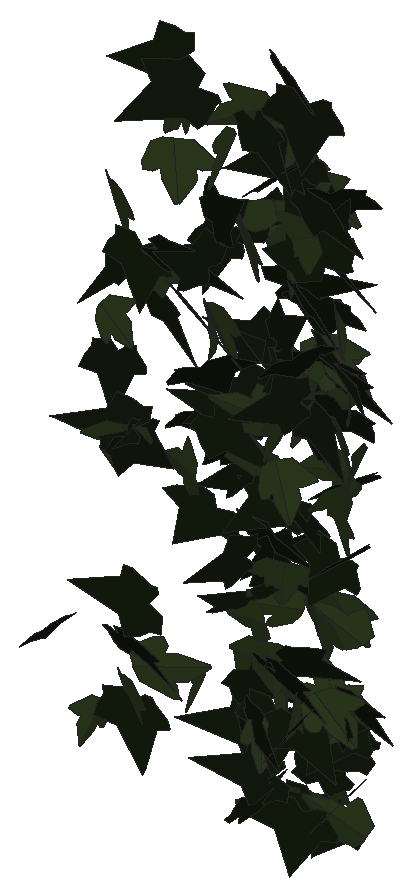
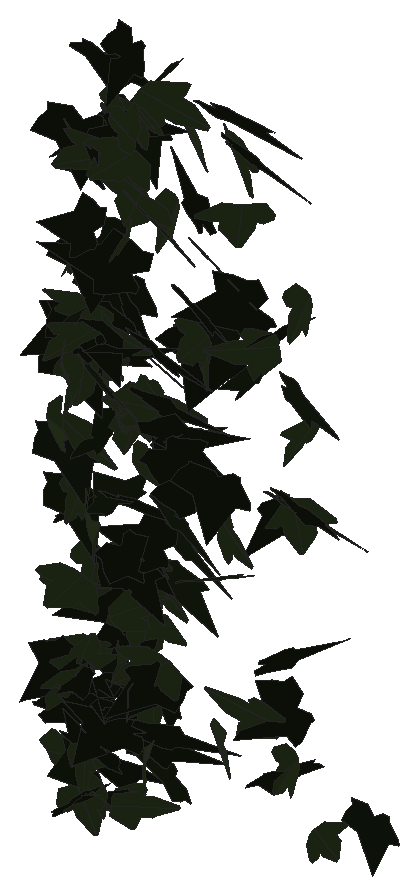
# SketchUp Ruby script. Lengths in inches.
U = 1.inch
M = Sketchup.active_model
def pt(a) = Geom::Point3d.new(a.map { |v| v * U })
def face(e, loops, mat)
  f = e.add_face(loops[0].map { |a| pt(a) })
  loops[1..].each { |l| e.add_face(l.map { |a| pt(a) }).erase! }
  f.material = f.back_material = mat if mat
  f
end
# faces: each face lists its corners as indices into pts; further lists are holes
def faces(e, pts, list, mat = nil) = list.each { |f| face(e, (f[0].is_a?(Array) ? f : [f]).map { |l| l.map { |i| pts[i] } }, mat) }
# xy, xz, yz: faces in a plane at the given z, y or x. An outline is a flat list of corners, or four numbers for a rectangle; further outlines are holes
def ring(l) = l.size == 4 ? [[l[0], l[1]], [l[2], l[1]], [l[2], l[3]], [l[0], l[3]]] : l.each_slice(2).to_a
def flat(e, list, mat, &to3) = list.each { |f| face(e, (f[0].is_a?(Array) ? f : [f]).map { |l| ring(l).map { |u, v| to3.(u, v) } }, mat) }
def xy(e, z, list, mat = nil) = flat(e, list, mat) { |x, y| [x, y, z] }
def xz(e, y, list, mat = nil) = flat(e, list, mat) { |x, z| [x, y, z] }
def yz(e, x, list, mat = nil) = flat(e, list, mat) { |y, z| [x, y, z] }
def lines(e, pts, list) = list.each { |a, b| e.add_line(pt(pts[a]), pt(pts[b])) }
# prism: a flat outline (further loops are holes) pulled along v
def prism(e, loops, v, mat = nil)
  f = face(e, loops, mat); d = Geom::Vector3d.new(v.map { |x| x * U })
  f.pushpull(f.normal.samedirection?(d) ? d.length : -d.length)
end
def box(e, o, s, mat = nil) = prism(e, [[o, [o[0] + s[0], o[1], o[2]], [o[0] + s[0], o[1] + s[1], o[2]], [o[0], o[1] + s[1], o[2]]]], [0, 0, s[2]], mat)
def at(x, y, z, deg = 0) = Geom::Transformation.translation(pt([x, y, z])) * Geom::Transformation.rotation(ORIGIN, Z_AXIS, deg.degrees)
def axes(o, x, y, z) = Geom::Transformation.new([*x, 0, *y, 0, *z, 0, *pt(o).to_a, 1])
def part(name) = M.definitions.add(name)
# library, detail: a bought-in or finely detailed component or shape, given as its bounding box
def library(name, o, s) = part(name).tap { |d| box(d.entities, o, s) }
def detail(e, o, s) = box(e.add_group.entities, o, s)
def put(e, d, t, mat = nil) = e.add_instance(d, t).tap { |i| i.material = mat if mat }
def group(e, t, mat = nil) = e.add_group.tap { |g| g.transformation = t; g.material = mat if mat }.entities
root = M.entities
M.materials.add("1026 AP 7946 SUNNY SIDE UP").color = [254, 231, 186]
M.materials.add("efeu1").color = [18, 25, 13]
M.materials.add("efeu2").color = [43, 57, 29]
c1 = part("ivyleaf_9")
p = [[1.54,2.16,1.25],[1.36,2.04,1.19],[-0.21,0.99,0.68],[-0.71,1.11,0.82],[-0.85,0.86,0.67],[-0.8,0.17,0.21],
  [-0.9,-0.01,0.1],[-0.67,-0.16,-0.02],[-0.08,-0.08,-0.05],[-0.03,-0.6,-0.4],[0.65,-0.88,-0.66],[0.83,-0.6,-0.49],
  [1.29,-0.42,-0.43],[1.8125,-0.07,-0.26],[1.21,0.44,0.15]]
faces(c1.entities,p,[[0,1,2,3,4,5,6,7,8,9,10,11,12,13,14]],"efeu1")
c2 = part("ivyleaf_10")
p = [[0,0.5,-0.03],[-0.0625,2.02,-0.43],[-0.19,2.01,-0.46],[-0.54,1.05,-0.29],[-0.52,0.625,-0.18],[-0.83,0.76,-0.28],
  [-1.16,0.64,-0.33],[-1.15,0.33,-0.24],[-0.77,-0.39,0.02],[-0.3,-0.51,0.16],[0.04,-0.48,0.23],[-0.02,2.01,-0.4375],
  [-0.06,2.01,-0.43],[0.04,-0.49,0.23],[0.67,-0.49,0.14],[1.38,0.36,-0.2],[1.375,0.51,-0.24],[0.81,0.65,-0.19],
  [0.62,0.59,-0.15],[0.6,1.09,-0.28],[0.5,1.23,-0.31]]
faces(c2.entities,p,[[0,1,2,3,4,5,6,7,8,9,10],[11,12,0,13,14,15,16,17,18,19,20]],"efeu2")
put(root,c1,axes([94.87,211.58,270.69],[-0.0572,-0.26498,-0.15518],[-0.0449,-0.13921,0.28391],[-0.50795,0.04214,-0.00762]),"1026 AP 7946 SUNNY SIDE UP")
put(root,c1,axes([96.16,211.21,274.97],[0.26752,0.28391,0.03135],[0.04691,0.01388,-0.34694],[-0.48162,0.15905,-0.01638]),"1026 AP 7946 SUNNY SIDE UP")
put(root,c1,axes([96.875,211.48,278.91],[0.18675,-0.28699,-0.05313],[-0.03244,0.04551,-0.31971],[0.4569,0.12054,-0.00098]),"1026 AP 7946 SUNNY SIDE UP")
put(root,c2,axes([96.35,211.52,278.41],[0.26232,-0.28547,0.07005],[0.03468,-0.06751,-0.34814],[0.4974,0.15525,-0.01267]),"1026 AP 7946 SUNNY SIDE UP")
put(root,c1,axes([94.69,211.55,269.06],[-0.08294,-0.28935,-0.03626],[0.01738,0.02879,-0.31371],[0.49353,-0.04964,0.00495]),"1026 AP 7946 SUNNY SIDE UP")
put(root,c1,axes([97.61,211.47,274.82],[-0.42003,0.15703,0.02672],[-0.06111,-0.01421,-0.31215],[-0.26236,-0.24809,0.02993]),"1026 AP 7946 SUNNY SIDE UP")
put(root,c2,axes([97.79,211.4,277.49],[0.28682,-0.1222,-0.23791],[-0.3066,0.12673,-0.22146],[0.29883,0.24732,0.00114]),"1026 AP 7946 SUNNY SIDE UP")
put(root,c1,axes([96.66,211.57,269.61],[-0.00932,-0.02444,-0.28773],[0.45485,-0.02975,-0.00338],[-0.04987,-0.26684,0.02293]),"1026 AP 7946 SUNNY SIDE UP")
put(root,c1,axes([96.77,211.32,268.17],[-0.13158,0.25409,-0.02418],[-0.00085,0.02692,0.28467],[0.43356,0.07717,-0.00678]),"1026 AP 7946 SUNNY SIDE UP")
put(root,c1,axes([96.08,211.58,277.08],[-0.0639,0.10843,0.29366],[0.11538,-0.26443,0.11883],[0.48493,0.07721,0.01042]),"1026 AP 7946 SUNNY SIDE UP")
put(root,c1,axes([95.54,211.58,275.66],[0.3356,-0.22608,0.10225],[0.09424,-0.08214,-0.32242],[0.40784,0.20501,-0.00963]),"1026 AP 7946 SUNNY SIDE UP")
put(root,c1,axes([96.66,211.49,272.05],[-0.37435,0.20551,-0.03339],[0.00764,-0.04462,-0.3218],[-0.35348,-0.2186,0.02841]),"1026 AP 7946 SUNNY SIDE UP")
put(root,c2,axes([97.29,211.49,273.59],[0.16217,0.30186,-0.00064],[0.01235,-0.00705,-0.33892],[-0.51232,0.09538,-0.00837]),"1026 AP 7946 SUNNY SIDE UP")
put(root,c1,axes([97.15,211.47,270.56],[0.47999,-0.06573,-0.02421],[-0.04383,-0.01521,-0.31021],[0.10905,0.28319,-0.01811]),"1026 AP 7946 SUNNY SIDE UP")
put(root,c1,axes([94.54,211.5,270.07],[0.49088,-0.09473,-0.00381],[-0.01982,-0.0282,-0.32453],[0.15964,0.2878,-0.02857]),"1026 AP 7946 SUNNY SIDE UP")
put(root,c1,axes([97.6,211.61,269.8125],[-0.21191,0.15107,-0.18646],[0.1486,-0.15458,-0.21051],[-0.36482,-0.15071,0.02257]),"1026 AP 7946 SUNNY SIDE UP")
put(root,c1,axes([97.01,211.65,268.72],[-0.16274,-0.11888,-0.22833],[-0.25336,-0.1507,0.16084],[-0.32514,0.17694,-0.01104]),"1026 AP 7946 SUNNY SIDE UP")
put(root,c1,axes([95.65,211.68,278.95],[-0.55344,0.00679,0.03369],[-0.05446,-0.05705,-0.34445],[-0.00201,-0.32252,0.057]),"1026 AP 7946 SUNNY SIDE UP")
put(root,c1,axes([96.03,211.4375,276.41],[-0.24336,0.21313,0.16311],[-0.16795,0.11336,-0.27285],[-0.40885,-0.17342,0.01499]),"1026 AP 7946 SUNNY SIDE UP")
put(root,c1,axes([97.51,211.69,268.27],[-0.34276,-0.16202,-0.10338],[0.16735,0.02637,-0.27368],[0.27083,-0.22135,0.03827]),"1026 AP 7946 SUNNY SIDE UP")
put(root,c1,axes([98.02,211.52,277.125],[-0.47997,-0.11707,0.04475],[0.05217,0.03868,0.32717],[-0.20538,0.28342,-0.02146]),"1026 AP 7946 SUNNY SIDE UP")
put(root,c2,axes([94.45,211.62,273.2],[-0.33009,-0.19302,0.04114],[-0.02393,-0.04388,-0.29319],[0.30937,-0.20935,0.02121]),"1026 AP 7946 SUNNY SIDE UP")
put(root,c2,axes([96.91,211.51,271.15],[-0.11736,0.04727,0.2582],[-0.39631,0.06361,-0.08432],[-0.12705,-0.24208,0.02452]),"1026 AP 7946 SUNNY SIDE UP")
put(root,c2,axes([97.38,211.75,269.89],[-0.02351,0.1138,-0.25251],[0.0071,-0.23755,-0.12551],[-0.44676,-0.00977,0.01129]),"1026 AP 7946 SUNNY SIDE UP")
put(root,c1,axes([97.6,211.4,275.52],[0.14076,0.31421,0.03727],[0.02603,0.02771,-0.34742],[-0.5353,0.08397,-0.00709]),"1026 AP 7946 SUNNY SIDE UP")
put(root,c1,axes([96.73,211.49,271.43],[-0.11108,0.29044,0.01419],[-0.18074,-0.01493,-0.29761],[-0.459,-0.06441,0.11375]),"1026 AP 7946 SUNNY SIDE UP")
put(root,c1,axes([97.74,211.55,278.03],[0.29979,-0.20789,-0.13977],[-0.07098,0.13771,-0.28442],[0.3828,0.18835,0.05672]),"1026 AP 7946 SUNNY SIDE UP")
put(root,c2,axes([94.52,211.62,269.27],[-0.28973,0.2273,-0.08865],[0.07086,-0.07582,-0.30511],[-0.40627,-0.17532,0.01]),"1026 AP 7946 SUNNY SIDE UP")
put(root,c2,axes([94.95,211.58,269.75],[0.1844,-0.04658,-0.29812],[0.47712,-0.00258,0.11806],[-0.03291,-0.29832,0.04126]),"1026 AP 7946 SUNNY SIDE UP")
put(root,c2,axes([96.88,211.64,269.4],[0.19198,0.23494,-0.06685],[-0.02787,-0.06471,-0.27971],[-0.4131,0.11355,-0.0122]),"1026 AP 7946 SUNNY SIDE UP")
put(root,c1,axes([97.29,211.47,278.26],[-0.02752,0.31474,0.00451],[-0.01167,-0.00025,-0.33732],[-0.53415,-0.01621,0.00714]),"1026 AP 7946 SUNNY SIDE UP")
put(root,c2,axes([96.99,211.64,270.65],[-0.49135,-0.04043,-0.00917],[0.02531,-0.04955,-0.30875],[0.06524,-0.28529,0.05075]),"1026 AP 7946 SUNNY SIDE UP")
put(root,c1,axes([97.4,211.49,270.71],[0.32388,0.10478,0.17347],[0.26949,0.04094,-0.22983],[-0.18277,0.24605,-0.03148]),"1026 AP 7946 SUNNY SIDE UP")
put(root,c2,axes([96.59,211.6,277.08],[-0.31685,0.26699,0.00127],[-0.01769,-0.01008,-0.34856],[-0.4529,-0.18639,0.01272]),"1026 AP 7946 SUNNY SIDE UP")
put(root,c1,axes([94.55,211.65,273.3],[-0.34071,0.18745,0.10444],[-0.23504,-0.01895,-0.27307],[-0.26847,-0.22129,0.10653]),"1026 AP 7946 SUNNY SIDE UP")
put(root,c1,axes([94.58,211.86,276],[-0.08138,-0.29026,0.03978],[-0.00215,-0.04064,-0.30392],[0.46077,-0.05145,0.0056]),"1026 AP 7946 SUNNY SIDE UP")
put(root,c1,axes([97.59,211.8,274.5],[0.13633,-0.28141,-0.04735],[-0.01116,0.04423,-0.30303],[0.44781,0.08677,0.00686]),"1026 AP 7946 SUNNY SIDE UP")
put(root,c1,axes([97.4,211.78,276.33],[0.33186,-0.21926,0.0085],[-0.01907,-0.02481,-0.31252],[0.34456,0.2098,-0.02549]),"1026 AP 7946 SUNNY SIDE UP")
put(root,c2,axes([93.78,211.89,268.53],[-0.09097,-0.2065,0.16072],[0.05963,-0.16604,-0.21132],[0.40369,-0.02201,0.06743]),"1026 AP 7946 SUNNY SIDE UP")
put(root,c1,axes([94.58,211.59,273.17],[0.04277,-0.07215,-0.30102],[-0.15559,0.26483,-0.07812],[0.46594,0.09506,0.00155]),"1026 AP 7946 SUNNY SIDE UP")
put(root,c1,axes([97.48,211.86,279.23],[-0.38777,-0.08938,-0.1823],[0.28106,0.03953,-0.26124],[0.16262,-0.28146,0.0168]),"1026 AP 7946 SUNNY SIDE UP")
put(root,c2,axes([96.62,211.91,278.9],[-0.17451,-0.10936,0.27038],[-0.26129,-0.20247,-0.16286],[0.38996,-0.18461,0.01187]),"1026 AP 7946 SUNNY SIDE UP")
put(root,c1,axes([96.01,211.72,273.88],[0.16498,-0.19799,-0.19559],[0.02213,0.20578,-0.21313],[0.42954,0.06544,0.08611]),"1026 AP 7946 SUNNY SIDE UP")
put(root,c2,axes([97.81,211.74,271.375],[-0.36683,0.1704,0.03418],[-0.06012,0.00295,-0.29384],[-0.2874,-0.21811,0.01783]),"1026 AP 7946 SUNNY SIDE UP")
put(root,c1,axes([97.28,212.01,278.3125],[-0.02011,-0.13612,-0.28715],[-0.07005,-0.26336,0.14233],[-0.50305,0.04211,-0.00834]),"1026 AP 7946 SUNNY SIDE UP")
put(root,c1,axes([97.35,211.79,269.65],[-0.00933,-0.22263,-0.19199],[0.03322,0.17575,-0.23562],[0.48107,-0.01645,0.01255]),"1026 AP 7946 SUNNY SIDE UP")
put(root,c2,axes([95.9,211.85,275.42],[-0.31982,0.17831,-0.15324],[0.1481,-0.11861,-0.27828],[-0.36146,-0.20636,0.02156]),"1026 AP 7946 SUNNY SIDE UP")
put(root,c1,axes([96.85,211.97,269.49],[-0.11786,-0.27392,0.03628],[-0.00549,-0.03781,-0.30298],[0.46929,-0.06924,0.00557]),"1026 AP 7946 SUNNY SIDE UP")
put(root,c2,axes([96.8,211.83,274.15],[0.02971,0.04397,0.29622],[-0.4508,-0.08395,0.03116],[0.1485,-0.26363,0.03532]),"1026 AP 7946 SUNNY SIDE UP")
put(root,c1,axes([94.82,211.89,275.34],[0.25126,-0.266,0.00567],[-0.01481,-0.01487,-0.32572],[0.45156,0.14752,-0.01384]),"1026 AP 7946 SUNNY SIDE UP")
put(root,c2,axes([95.31,211.81,278.64],[0.35807,-0.23526,-0.07977],[-0.05241,0.06805,-0.33651],[0.41406,0.21205,0.02639]),"1026 AP 7946 SUNNY SIDE UP")
put(root,c1,axes([95.03,211.75,276.16],[0.44767,-0.01306,0.13588],[0.21159,-0.03769,-0.28157],[0.04761,0.29031,-0.02631]),"1026 AP 7946 SUNNY SIDE UP")
put(root,c1,axes([97.86,212.02,272.22],[-0.18738,-0.22591,0.12511],[-0.07553,-0.11154,-0.27059],[0.42746,-0.11874,0.00703]),"1026 AP 7946 SUNNY SIDE UP")
put(root,c2,axes([97.03,211.96,274.12],[0.01257,-0.27508,0.1221],[0.0089,-0.11754,-0.29623],[0.50779,0.00887,0.00217]),"1026 AP 7946 SUNNY SIDE UP")
put(root,c2,axes([95.13,211.9,277.6875],[0.35159,0.24137,-0.00952],[0.01466,-0.02323,-0.34003],[-0.40998,0.20616,-0.02032]),"1026 AP 7946 SUNNY SIDE UP")
put(root,c1,axes([96.88,211.96,275.34],[-0.04376,0.13452,0.26061],[0.08835,-0.23603,0.1433],[0.46115,0.05799,-0.00273]),"1026 AP 7946 SUNNY SIDE UP")
put(root,c2,axes([98.26,211.89,268.22],[0.16626,0.04869,0.27723],[-0.41598,-0.05371,0.1169],[0.10724,-0.28384,0.02367]),"1026 AP 7946 SUNNY SIDE UP")
put(root,c1,axes([96.63,211.98,269.16],[-0.34558,0.03431,0.20913],[-0.33583,-0.04189,-0.21393],[0.00794,-0.2787,0.05386]),"1026 AP 7946 SUNNY SIDE UP")
put(root,c2,axes([97.0625,211.96,278.65],[0.49124,-0.1076,-0.00905],[-0.02698,-0.02259,-0.32961],[0.18105,0.28858,-0.02456]),"1026 AP 7946 SUNNY SIDE UP")
put(root,c1,axes([97.94,211.81,278.03],[0.26433,0.2174,-0.09943],[-0.07674,-0.08523,-0.28718],[-0.39586,0.16169,-0.01073]),"1026 AP 7946 SUNNY SIDE UP")
put(root,c2,axes([97.95,211.94,276.15],[-0.09297,0.24904,-0.10713],[0.015,-0.10371,-0.2741],[-0.45744,-0.05401,0.01278]),"1026 AP 7946 SUNNY SIDE UP")
put(root,c2,axes([97.8,211.81,270.02],[0.22653,0.22464,0.14483],[0.14112,0.10427,-0.27774],[-0.41951,0.15638,-0.01522]),"1026 AP 7946 SUNNY SIDE UP")
put(root,c2,axes([96.82,211.95,277.3],[0.47525,0.00646,0.13538],[0.21479,-0.01186,-0.29962],[-0.00171,0.30693,-0.01014]),"1026 AP 7946 SUNNY SIDE UP")
put(root,c2,axes([96.62,212.09,268.72],[-0.03832,-0.04977,0.27401],[0.27202,-0.20857,-0.02507],[0.32774,0.16729,0.05285]),"1026 AP 7946 SUNNY SIDE UP")
put(root,c2,axes([95.5,211.96,269.52],[0.17485,-0.24806,-0.0299],[-0.02263,0.02381,-0.27989],[0.39181,0.11208,-0.00282]),"1026 AP 7946 SUNNY SIDE UP")
put(root,c2,axes([97,211.95,271.79],[-0.38451,-0.1389,0.01884],[-0.00762,-0.02967,-0.28382],[0.23796,-0.2254,0.02135]),"1026 AP 7946 SUNNY SIDE UP")
put(root,c2,axes([97.01,212.03,276.75],[-0.05174,0.24448,-0.14537],[0.02759,-0.13803,-0.26569],[-0.47659,-0.03453,0.0004]),"1026 AP 7946 SUNNY SIDE UP")
put(root,c1,axes([98.06,211.85,272.34],[-0.0356,0.29961,-0.01229],[-0.00722,-0.01571,-0.32171],[-0.50921,-0.02072,0.00542]),"1026 AP 7946 SUNNY SIDE UP")
put(root,c2,axes([96.52,211.98,270.24],[-0.37481,0.0011,-0.19532],[0.30659,-0.0394,-0.23479],[-0.04403,-0.28371,0.02782]),"1026 AP 7946 SUNNY SIDE UP")
put(root,c2,axes([97.44,211.92,275],[0.14514,0.03295,0.29053],[-0.46036,0.04236,0.0867],[-0.05239,-0.28094,0.04308]),"1026 AP 7946 SUNNY SIDE UP")
put(root,c1,axes([97.63,211.92,276.22],[0.36179,0.09962,-0.15688],[-0.21528,-0.07721,-0.25251],[-0.21268,0.24762,-0.01127]),"1026 AP 7946 SUNNY SIDE UP")
put(root,c1,axes([96.35,212.09,273.86],[-0.17951,0.01615,0.28327],[-0.44795,-0.03108,-0.1114],[0.03894,-0.28305,0.02438]),"1026 AP 7946 SUNNY SIDE UP")
put(root,c1,axes([97.03,212.18,272.68],[0.00517,-0.23854,0.16513],[0.16942,-0.14891,-0.22952],[0.42022,0.06297,0.0905]),"1026 AP 7946 SUNNY SIDE UP")
put(root,c2,axes([94.03,211.97,276.68],[-0.33148,0.23888,-0.02669],[0.00876,-0.03195,-0.33031],[-0.4082,-0.19467,0.01458]),"1026 AP 7946 SUNNY SIDE UP")
put(root,c1,axes([97.7,212.14,275.36],[0.14803,-0.25542,0.09314],[0.04919,-0.08556,-0.29014],[0.45727,0.09189,0.00106]),"1026 AP 7946 SUNNY SIDE UP")
put(root,c1,axes([96.63,212.03,274.3],[-0.33025,0.08397,0.17656],[-0.2874,0.01201,-0.22166],[-0.12275,-0.25405,0.04394]),"1026 AP 7946 SUNNY SIDE UP")
put(root,c1,axes([97.02,211.93,279.59],[0.39592,-0.0887,-0.18989],[-0.29397,0.03864,-0.26567],[0.1604,0.28975,-0.01821]),"1026 AP 7946 SUNNY SIDE UP")
put(root,c1,axes([96.39,212.07,272.14],[0.2757,-0.11738,0.19712],[0.23972,-0.1171,-0.21784],[0.2603,0.23216,-0.00817]),"1026 AP 7946 SUNNY SIDE UP")
put(root,c2,axes([96.5625,212,273.24],[-0.40637,0.02517,-0.11763],[-0.17797,0.04709,0.25598],[0.07177,0.2593,-0.0313]),"1026 AP 7946 SUNNY SIDE UP")
put(root,c2,axes([95.86,211.81,275.16],[0.05365,-0.04456,-0.31393],[-0.13999,0.28134,-0.05147],[0.48262,0.08656,0.01997]),"1026 AP 7946 SUNNY SIDE UP")
put(root,c2,axes([96.93,212.16,268.04],[0.03393,0.00682,-0.28081],[-0.35571,-0.15226,-0.02326],[-0.23945,0.22716,-0.00523]),"1026 AP 7946 SUNNY SIDE UP")
put(root,c2,axes([93.97,211.91,274.75],[0.01621,0.26047,0.13239],[0.01722,0.12667,-0.26774],[-0.45534,0.01406,-0.00541]),"1026 AP 7946 SUNNY SIDE UP")
put(root,c1,axes([97.3,212.09,274.79],[-0.31288,-0.18546,-0.08653],[-0.11904,-0.04052,0.27852],[-0.3204,0.19616,-0.01898]),"1026 AP 7946 SUNNY SIDE UP")
put(root,c1,axes([96.9,212.18,272.75],[-0.48087,-0.0407,0.02803],[-0.02805,-0.06799,-0.29941],[0.07775,-0.27629,0.06537]),"1026 AP 7946 SUNNY SIDE UP")
put(root,c2,axes([97.27,212.1,274.3],[0.28181,-0.23521,-0.00339],[-0.00747,-0.00116,-0.30461],[0.36978,0.17923,-0.00357]),"1026 AP 7946 SUNNY SIDE UP")
put(root,c1,axes([95.86,212.04,273.1],[0.25349,0.21839,0.07129],[-0.08189,-0.04412,0.28219],[0.37741,-0.15625,0.01335]),"1026 AP 7946 SUNNY SIDE UP")
put(root,c1,axes([97.9375,212.02,274.59],[0.20709,0.10435,-0.22744],[-0.32048,-0.10375,-0.17098],[-0.24576,0.22322,0.03132]),"1026 AP 7946 SUNNY SIDE UP")
put(root,c2,axes([97.03,211.89,269.59],[-0.02702,0.13834,-0.23153],[-0.04104,0.21672,0.15211],[0.43646,0.02894,-0.00003]),"1026 AP 7946 SUNNY SIDE UP")
put(root,c2,axes([94.73,211.9,275.71],[-0.01839,-0.0284,-0.32471],[0.3897,0.19817,-0.02591],[0.33896,-0.22937,0.01217]),"1026 AP 7946 SUNNY SIDE UP")
put(root,c1,axes([97.69,211.98,275.25],[0.19249,0.2079,-0.19575],[-0.30977,-0.09601,-0.23588],[-0.35751,0.19512,0.09898]),"1026 AP 7946 SUNNY SIDE UP")
put(root,c1,axes([96.72,211.93,277.09],[-0.15706,0.20871,0.18785],[-0.1851,0.13841,-0.23962],[-0.421,-0.13872,0.03528]),"1026 AP 7946 SUNNY SIDE UP")
put(root,c1,axes([95.49,212.3,272.06],[-0.32868,-0.16914,0.11492],[0.00176,-0.15275,-0.25266],[0.34208,-0.16173,0.11172]),"1026 AP 7946 SUNNY SIDE UP")
put(root,c2,axes([97.9,212.04,273.27],[-0.15535,-0.26226,-0.08211],[0.05406,0.06647,-0.29633],[0.45908,-0.09657,0.00711]),"1026 AP 7946 SUNNY SIDE UP")
put(root,c1,axes([97.84,211.93,277.54],[0.10907,-0.00564,0.29408],[-0.12072,0.27222,0.02759],[-0.45064,-0.07429,0.06379]),"1026 AP 7946 SUNNY SIDE UP")
put(root,c2,axes([96.875,212.25,271.03],[0.03264,0.08707,0.27115],[-0.08078,-0.24762,0.09198],[0.44555,-0.05127,-0.00319]),"1026 AP 7946 SUNNY SIDE UP")
put(root,c1,axes([96.47,211.92,270.04],[0.00955,-0.05325,-0.30544],[-0.02874,0.28411,-0.05331],[0.49068,0.01768,0.00282]),"1026 AP 7946 SUNNY SIDE UP")
put(root,c2,axes([97.64,212.08,275.42],[0.3649,0.11215,0.14472],[0.22574,0.03213,-0.25726],[-0.19186,0.2511,-0.02745]),"1026 AP 7946 SUNNY SIDE UP")
put(root,c1,axes([97.9,212.01,269.83],[0.07164,-0.01072,-0.2746],[-0.4342,0.01864,-0.04565],[0.0342,0.25913,-0.00443]),"1026 AP 7946 SUNNY SIDE UP")
put(root,c2,axes([95.36,211.97,272.72],[-0.03323,0.04019,0.31252],[-0.43998,0.13573,-0.03679],[-0.23611,-0.25859,0.02457]),"1026 AP 7946 SUNNY SIDE UP")
put(root,c1,axes([96.6,212.04,275.11],[-0.21159,0.15498,0.19995],[-0.25951,0.11005,-0.20772],[-0.31658,-0.1938,0.03663]),"1026 AP 7946 SUNNY SIDE UP")
put(root,c1,axes([97.22,212.27,268.12],[-0.19521,-0.22659,-0.00095],[0.025,-0.00913,-0.26555],[0.35541,-0.12381,0.01816]),"1026 AP 7946 SUNNY SIDE UP")
put(root,c2,axes([97.35,212.07,277.85],[0.2606,0.09046,0.25374],[0.35681,0.10729,-0.18905],[-0.23778,0.26015,-0.00559]),"1026 AP 7946 SUNNY SIDE UP")
put(root,c2,axes([97.8125,212.1,274.26],[-0.23491,0.26198,-0.0102],[-0.00841,-0.01724,-0.31716],[-0.44519,-0.13791,0.01137]),"1026 AP 7946 SUNNY SIDE UP")
put(root,c2,axes([96.72,211.97,274.15],[-0.02371,-0.11625,0.26634],[0.07212,0.24673,0.12866],[-0.4629,0.0444,0.00641]),"1026 AP 7946 SUNNY SIDE UP")
put(root,c1,axes([97.7,212.08,275.06],[0.45987,-0.01551,0.03861],[0.05852,-0.02918,-0.28948],[0.03254,0.27176,-0.02503]),"1026 AP 7946 SUNNY SIDE UP")
put(root,c1,axes([94.02,212.23,275.46],[-0.35203,0.12132,-0.14137],[0.14258,-0.11609,-0.25753],[-0.25117,-0.23594,0.05194]),"1026 AP 7946 SUNNY SIDE UP")
put(root,c2,axes([97.62,212.14,274.61],[-0.29085,-0.22046,-0.06344],[0.08123,0.0341,-0.29791],[0.37764,-0.17712,0.01522]),"1026 AP 7946 SUNNY SIDE UP")
put(root,c2,axes([97.35,212.34,272.06],[-0.0687,0.0305,-0.26343],[0.03705,-0.2483,-0.0402],[-0.41993,-0.0269,0.03955]),"1026 AP 7946 SUNNY SIDE UP")
put(root,c1,axes([96.96,212.06,276.18],[0.17132,0.00473,0.29646],[0.46794,0.02611,-0.10769],[-0.04439,0.29351,0.00894]),"1026 AP 7946 SUNNY SIDE UP")
put(root,c1,axes([97.78,211.93,268.23],[-0.14367,0.20051,-0.18517],[-0.12944,0.16119,0.22785],[0.4044,0.12282,0.00714]),"1026 AP 7946 SUNNY SIDE UP")
put(root,c2,axes([97.81,212.35,274.62],[0.04437,-0.02204,0.29192],[0.2796,-0.21779,-0.03875],[0.37138,0.1666,-0.0057]),"1026 AP 7946 SUNNY SIDE UP")
put(root,c1,axes([97.17,212,269.2],[0.32516,0.19581,0.07057],[0.09039,0.03647,-0.29245],[-0.33747,0.19843,-0.01033]),"1026 AP 7946 SUNNY SIDE UP")
put(root,c1,axes([97.74,212.32,269.46],[-0.36036,-0.16443,0.00711],[0.00968,-0.02167,-0.28692],[0.27935,-0.21135,0.01912]),"1026 AP 7946 SUNNY SIDE UP")
put(root,c1,axes([97.43,212.27,276.75],[0.28985,-0.18355,0.13513],[0.11607,-0.11132,-0.26881],[0.36233,0.1825,-0.02199]),"1026 AP 7946 SUNNY SIDE UP")
put(root,c1,axes([96.85,212.27,272.0625],[-0.04728,0.1341,-0.24922],[0.02071,-0.23491,-0.14862],[-0.45815,-0.02446,0.019]),"1026 AP 7946 SUNNY SIDE UP")
put(root,c2,axes([97.7,212.12,269.93],[0.24328,0.23654,-0.00275],[-0.03037,0.01741,0.29008],[0.37075,-0.15379,0.02557]),"1026 AP 7946 SUNNY SIDE UP")
put(root,c1,axes([96.91,212.17,271.74],[0.15583,0.06042,-0.24528],[-0.33057,-0.1222,-0.11934],[-0.23138,0.21528,0.0053]),"1026 AP 7946 SUNNY SIDE UP")
put(root,c2,axes([97.96,212.21,271],[0.23166,0.0784,0.22472],[-0.34387,-0.0591,0.1646],[0.15875,-0.24241,0.02861]),"1026 AP 7946 SUNNY SIDE UP")
put(root,c1,axes([97.47,212.14,268.61],[-0.26674,0.13536,0.1508],[0.18478,-0.08671,0.22077],[0.27278,0.1911,-0.00209]),"1026 AP 7946 SUNNY SIDE UP")
put(root,c2,axes([97.38,212.23,268.16],[-0.30562,0.14635,-0.09237],[0.08201,-0.07998,-0.24914],[-0.25783,-0.19892,0.03024]),"1026 AP 7946 SUNNY SIDE UP")
put(root,c1,axes([98.09,212.32,269.18],[-0.21717,-0.15508,-0.12616],[-0.05755,-0.11873,0.20864],[-0.3235,0.12523,0.04758]),"1026 AP 7946 SUNNY SIDE UP")
put(root,c2,axes([97.82,212.1875,273.51],[-0.16457,0.05806,0.2676],[-0.43375,-0.00788,-0.10456],[-0.02296,-0.26728,0.0573]),"1026 AP 7946 SUNNY SIDE UP")
put(root,c2,axes([96.875,212.22,278.06],[-0.40493,0.00335,-0.171],[0.26659,-0.04819,-0.25278],[-0.05019,-0.28303,0.03695]),"1026 AP 7946 SUNNY SIDE UP")
put(root,c2,axes([96.68,212.35,278.52],[-0.09808,-0.02081,0.295],[0.4277,-0.12025,0.04511],[0.19379,0.25487,0.04974]),"1026 AP 7946 SUNNY SIDE UP")
put(root,c1,axes([97.62,212.44,267.95],[-0.16015,-0.21129,0.14251],[-0.08401,-0.12908,-0.2423],[0.38918,-0.11481,0.00634]),"1026 AP 7946 SUNNY SIDE UP")
put(root,c2,axes([97.9375,212.41,273.6875],[0.13847,-0.16617,0.2075],[0.1214,-0.18281,-0.20036],[0.41895,0.1079,-0.01052]),"1026 AP 7946 SUNNY SIDE UP")
put(root,c2,axes([97.86,212.375,269.6],[0.105,0.12798,-0.20834],[-0.15514,-0.17374,-0.15455],[-0.36625,0.11028,0.00574]),"1026 AP 7946 SUNNY SIDE UP")
put(root,c1,axes([93.74,212.38,273.84],[-0.29763,-0.09727,-0.1912],[0.31719,-0.01946,-0.20215],[0.08628,-0.26399,0.08359]),"1026 AP 7946 SUNNY SIDE UP")
put(root,c1,axes([92.7,212.1,269.28],[0.03884,0.25805,0.05512],[0.01969,0.05105,-0.26665],[-0.41346,0.02668,-0.00752]),"1026 AP 7946 SUNNY SIDE UP")
put(root,c1,axes([97.14,212.29,273.82],[0.30809,-0.17814,-0.06246],[-0.09222,0.02438,-0.27106],[0.3033,0.18837,-0.01896]),"1026 AP 7946 SUNNY SIDE UP")
put(root,c1,axes([96.15,212.23,272.92],[-0.3048,0.22356,0.01311],[-0.02634,-0.00051,-0.30669],[-0.37891,-0.1798,0.01078]),"1026 AP 7946 SUNNY SIDE UP")
put(root,c1,axes([97.9,212.17,273.34],[0.03455,0.28631,-0.04057],[-0.03246,-0.04031,-0.30737],[-0.49005,0.02285,0.0175]),"1026 AP 7946 SUNNY SIDE UP")
put(root,c2,axes([97.68,212.31,269.86],[0.16803,0.24919,-0.05156],[-0.0088,-0.05318,-0.28737],[-0.43182,0.09805,-0.0142]),"1026 AP 7946 SUNNY SIDE UP")
put(root,c1,axes([95.57,212.41,276.33],[-0.36219,-0.01273,-0.19366],[0.30331,-0.06102,-0.22207],[-0.05093,-0.27288,0.05469]),"1026 AP 7946 SUNNY SIDE UP")
put(root,c1,axes([94.9,212.27,278.9],[-0.36926,0.1531,0.12215],[-0.17635,0.04273,-0.28754],[-0.24719,-0.25919,0.02266]),"1026 AP 7946 SUNNY SIDE UP")
put(root,c1,axes([95.35,212.14,273.59],[0.1709,0.27279,0.00685],[0.02794,-0.00305,-0.31084],[-0.46226,0.10067,-0.01625]),"1026 AP 7946 SUNNY SIDE UP")
put(root,c1,axes([95.9375,212.4375,273.94],[-0.00822,0.03518,-0.28341],[-0.06889,-0.26226,-0.04012],[-0.44885,0.03961,0.01135]),"1026 AP 7946 SUNNY SIDE UP")
put(root,c2,axes([97.6,212.25,268.61],[-0.30954,0.14021,0.10404],[-0.14833,0.03962,-0.24783],[-0.22676,-0.2173,0.02009]),"1026 AP 7946 SUNNY SIDE UP")
put(root,c1,axes([97.74,212.26,269.96],[0.46429,-0.01327,-0.01983],[-0.03234,-0.01461,-0.29289],[0.02079,0.27373,-0.01276]),"1026 AP 7946 SUNNY SIDE UP")
put(root,c2,axes([97.57,212.34,268.02],[-0.35257,0.00013,0.10988],[-0.17251,-0.03275,-0.22057],[0.02443,-0.22935,0.02829]),"1026 AP 7946 SUNNY SIDE UP")
put(root,c1,axes([97.33,212.4,274.7],[-0.37276,0.11615,-0.08351],[0.09661,-0.06152,-0.26529],[-0.21855,-0.2253,0.02517]),"1026 AP 7946 SUNNY SIDE UP")
put(root,c2,axes([97.59,212.34,272.72],[-0.29871,0.20252,-0.03621],[0.01757,-0.03921,-0.28714],[-0.34887,-0.17538,0.01655]),"1026 AP 7946 SUNNY SIDE UP")
put(root,c2,axes([97.59,212.23,275.08],[0.1394,0.19497,0.19415],[0.15065,0.15608,-0.22364],[-0.42306,0.11982,-0.01566]),"1026 AP 7946 SUNNY SIDE UP")
put(root,c2,axes([97.64,212.37,271.32],[-0.41868,0.03424,-0.12259],[0.18452,-0.04732,-0.26543],[-0.08609,-0.26797,0.02729]),"1026 AP 7946 SUNNY SIDE UP")
